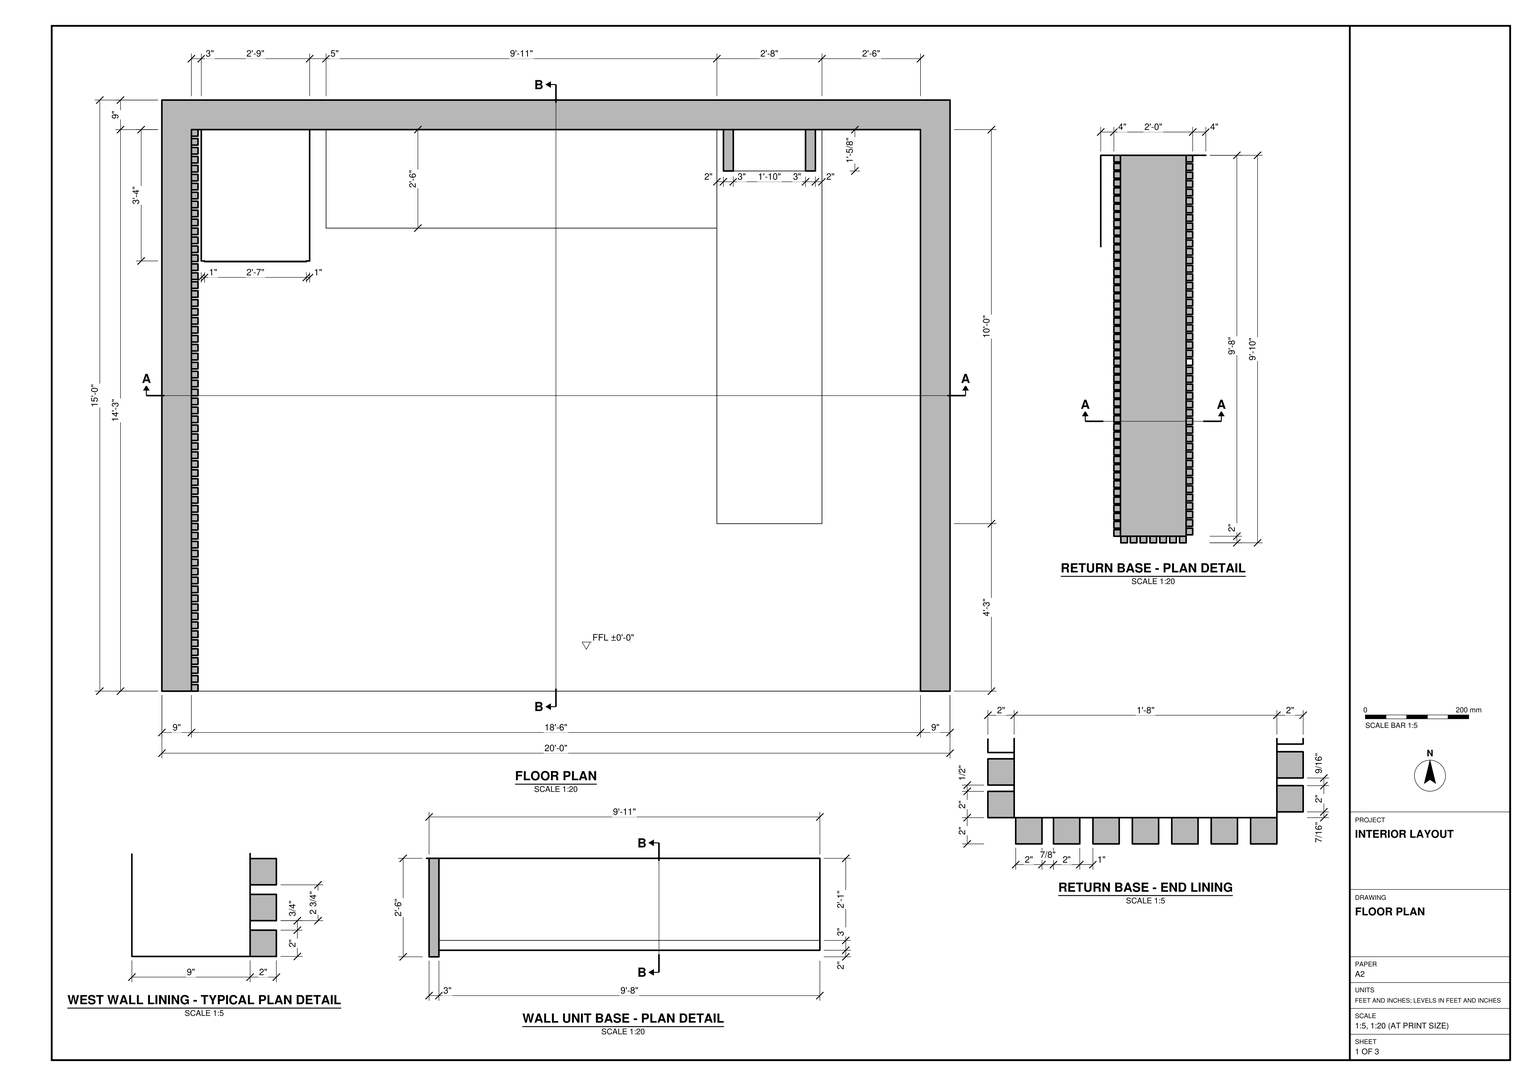
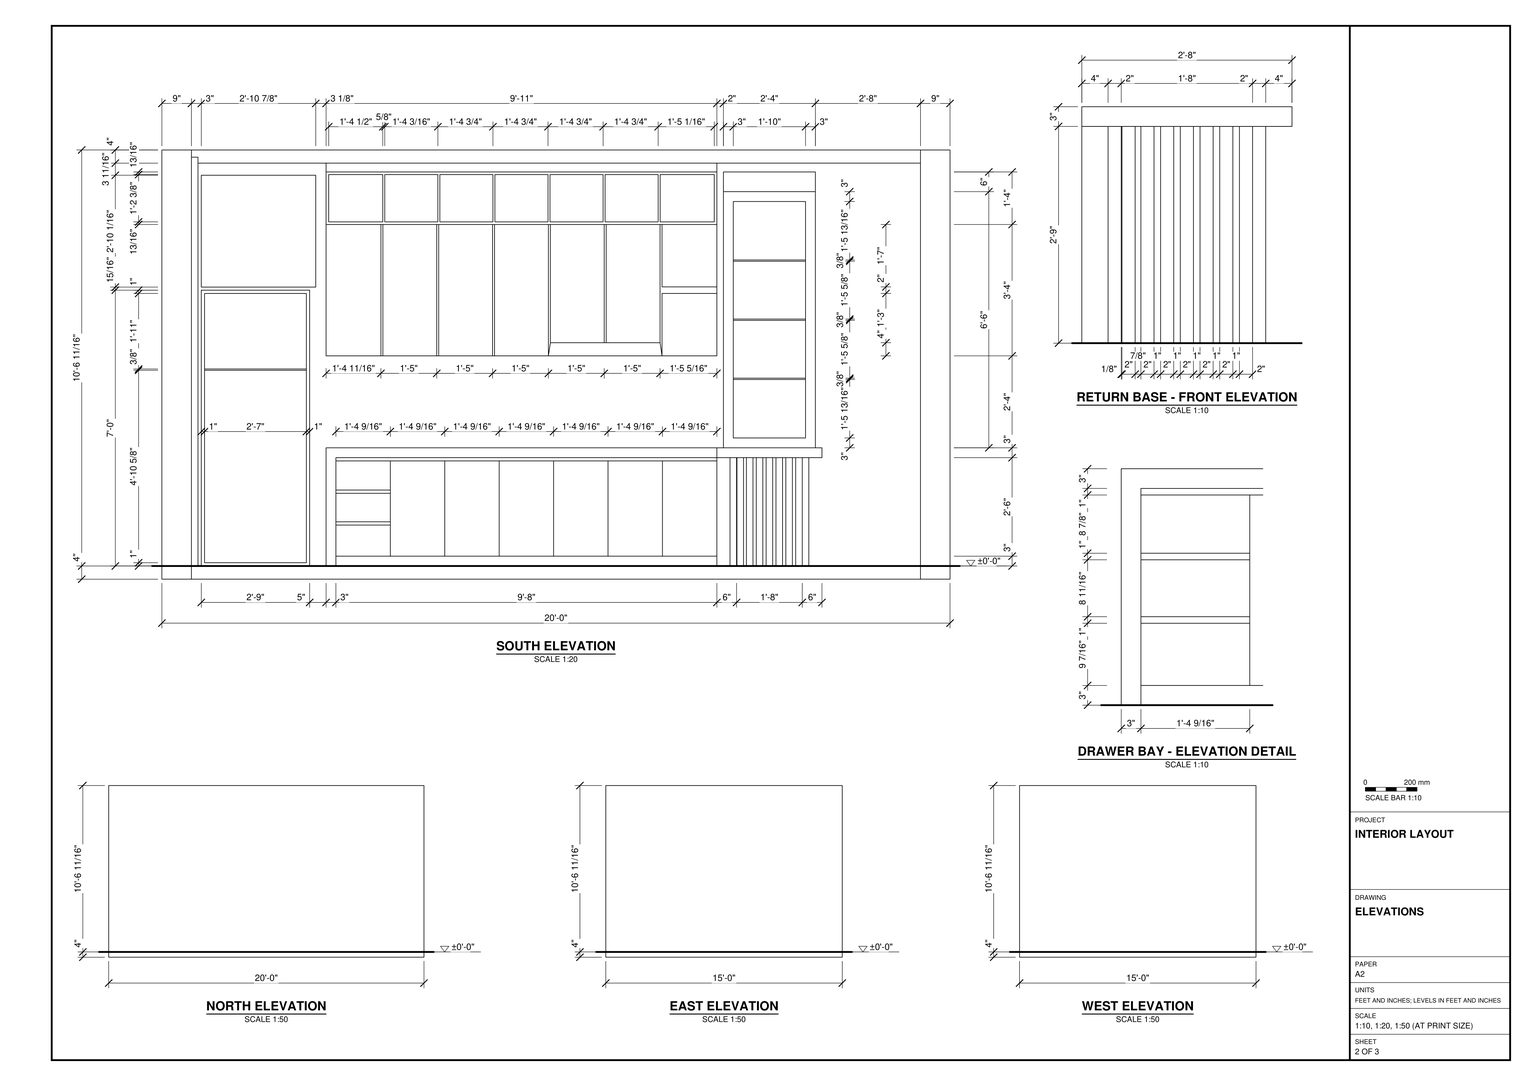
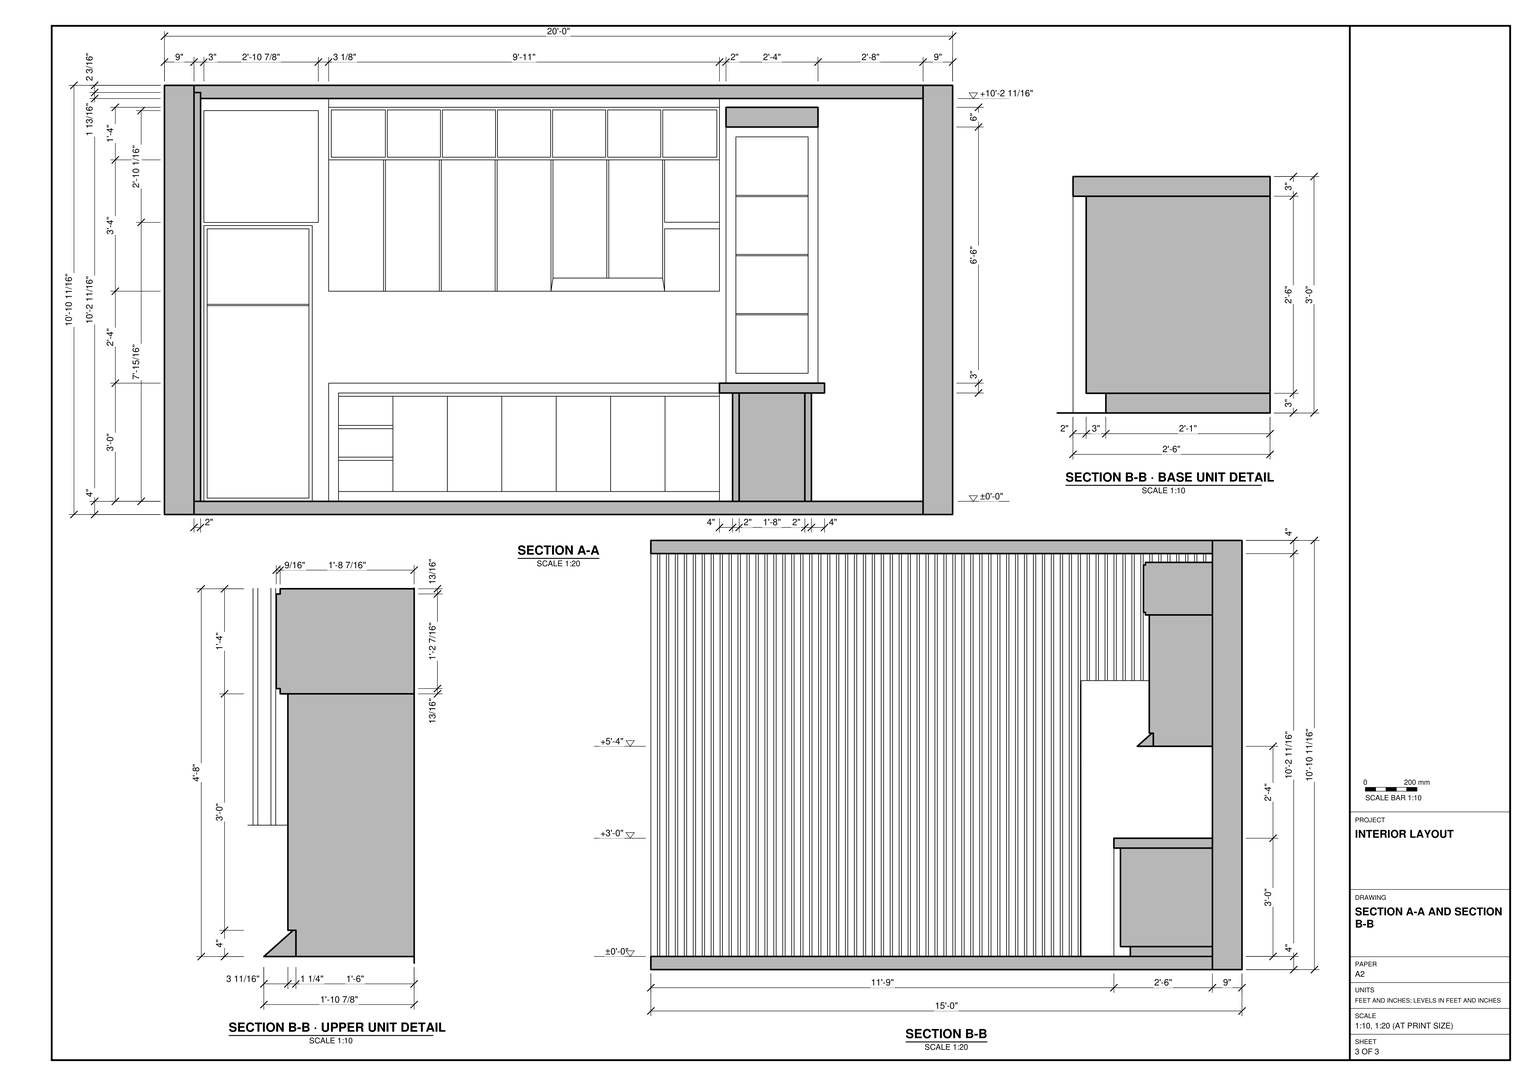
Build the single-level kitchen interior in SketchUp from task_files/diagram_01.pdf. Work in feet and inches. Set the finished floor at ±0'-0" and make the overall model 20'-0" wide, 15'-0" deep and 10'-10 11/16" high. Model the floor and overhead slabs, the 9" back and side walls, and the open front shown in plan. Line the inside of the west wall with the spaced vertical strips shown in the plan detail and section.

Use the south elevation to lay out the back wall. Place the tall unit and its overhead cupboard at the west end. Beside them, build the base cabinets with a drawer bay, divided fronts, a recessed plinth and a projecting countertop. Model the cupboards above the work surface in two tiers, following the changes in depth and lower-edge profile shown in section. At the right end, turn the counter into the room. Set its top over a narrower base with vertical strips along both sides and around the exposed end. Place the narrow shelving unit above the counter where the return meets the back wall.

Keep shell elements and each furniture or joinery piece in separate groups or components. Use components for repeated parts such as lining strips and cabinet fronts. Decor and loose items may be any suitable library components. Save one SketchUp model as output_files/kitchen_interior_with_a_slatted_counter_return.skp.

# SketchUp Ruby script. Lengths in inches.
U = 1.inch
M = Sketchup.active_model
def pt(a) = Geom::Point3d.new(a.map { |v| v * U })
def face(e, loops, mat)
  f = e.add_face(loops[0].map { |a| pt(a) })
  loops[1..].each { |l| e.add_face(l.map { |a| pt(a) }).erase! }
  f.material = f.back_material = mat if mat
  f
end
# faces: each face lists its corners as indices into pts; further lists are holes
def faces(e, pts, list, mat = nil) = list.each { |f| face(e, (f[0].is_a?(Array) ? f : [f]).map { |l| l.map { |i| pts[i] } }, mat) }
# xy, xz, yz: faces in a plane at the given z, y or x. An outline is a flat list of corners, or four numbers for a rectangle; further outlines are holes
def ring(l) = l.size == 4 ? [[l[0], l[1]], [l[2], l[1]], [l[2], l[3]], [l[0], l[3]]] : l.each_slice(2).to_a
def flat(e, list, mat, &to3) = list.each { |f| face(e, (f[0].is_a?(Array) ? f : [f]).map { |l| ring(l).map { |u, v| to3.(u, v) } }, mat) }
def xy(e, z, list, mat = nil) = flat(e, list, mat) { |x, y| [x, y, z] }
def xz(e, y, list, mat = nil) = flat(e, list, mat) { |x, z| [x, y, z] }
def yz(e, x, list, mat = nil) = flat(e, list, mat) { |y, z| [x, y, z] }
def lines(e, pts, list) = list.each { |a, b| e.add_line(pt(pts[a]), pt(pts[b])) }
# prism: a flat outline (further loops are holes) pulled along v
def prism(e, loops, v, mat = nil)
  f = face(e, loops, mat); d = Geom::Vector3d.new(v.map { |x| x * U })
  f.pushpull(f.normal.samedirection?(d) ? d.length : -d.length)
end
def box(e, o, s, mat = nil) = prism(e, [[o, [o[0] + s[0], o[1], o[2]], [o[0] + s[0], o[1] + s[1], o[2]], [o[0], o[1] + s[1], o[2]]]], [0, 0, s[2]], mat)
def at(x, y, z, deg = 0) = Geom::Transformation.translation(pt([x, y, z])) * Geom::Transformation.rotation(ORIGIN, Z_AXIS, deg.degrees)
def axes(o, x, y, z) = Geom::Transformation.new([*x, 0, *y, 0, *z, 0, *pt(o).to_a, 1])
def part(name) = M.definitions.add(name)
# library, detail: a bought-in or finely detailed component or shape, given as its bounding box
def library(name, o, s) = part(name).tap { |d| box(d.entities, o, s) }
def detail(e, o, s) = box(e.add_group.entities, o, s)
def put(e, d, t, mat = nil) = e.add_instance(d, t).tap { |i| i.material = mat if mat }
def group(e, t, mat = nil) = e.add_group.tap { |g| g.transformation = t; g.material = mat if mat }.entities
root = M.entities
M.materials.add("[0007_MistyRose]").color = [255, 228, 225]
M.materials.add("[0035_Tan]").color = [210, 180, 140]
M.materials.add("[0042_Sienna]").color = [160, 82, 45]
M.materials.add("[0043_SaddleBrown]").color = [139, 69, 19]
M.materials.add("[0131_Silver]").color = [192, 192, 192]
M.materials.add("[0134_DimGray]").color = [105, 105, 105]
M.materials.add("[0135_DarkGray]").color = [81, 81, 81]
M.materials.add("[0137_Black]").color = [0, 0, 0]
M.materials.add("[Carrera Marble]").color = [244, 244, 244]
M.materials.add("[Carrera Marble]1").color = [237, 237, 237]
M.materials.add("[Carrera Marble]2").color = [207, 207, 207]
M.materials.add("[Terrazzo Tile Accent]").color = [224, 221, 217]
M.materials.add("[Tile Various Tan]").color = [214, 196, 169]
M.materials.add("[Wood Bamboo]").color = [177, 105, 43]
c1 = part("Vertical timber slat")
box(c1.entities,[0,0,0],[2,2,124.5],"[Wood Bamboo]")
c2 = part("Horizontal counter slat")
box(c2.entities,[0,0,0],[2,33,2],"[Wood Bamboo]")
xy(root,-4,[[0,0,0,180,240,180,240,0,231,0,231,171,9,171,9,0]])
xy(root,0,[[12,131,45,171]])
xy(root,1,[[13,130.8,44,131]])
xy(root,59.6,[[13,130.8,44,131]])
xy(root,60,[[13,130.8,44,131]])
xy(root,64,[[117.7,148.11,152.3,153]],"[0135_DarkGray]")
xy(root,68,[[118.3,152.59,151.7,153]])
xy(root,83,[[13,130.8,44,131]])
xy(root,84,[[12,131,45,171]],"[0134_DimGray]")
xy(root,104,[[50,150.6,169,171]])
xy(root,104.8,[[50.8,150,67.27,150.6],[67.87,150,84.04,150.6],[84.64,150,100.8125,150.6],[101.41,150,117.59,150.6],[118.1875,150,134.36,150.6],
  [134.96,150,151.13,150.6],[151.73,150,168.2,150.6]])
xy(root,119.2,[[50.8,150,67.27,150.6],[67.87,150,84.04,150.6],[84.64,150,100.8125,150.6],[101.41,150,117.59,150.6],[118.1875,150,134.36,150.6],
  [134.96,150,151.13,150.6],[151.73,150,168.2,150.6]])
xy(root,120,[[50,150.6,169,171]])
xy(root,126.6875,[[0,0,9,0,9,171,231,171,231,0,240,0,240,180,0,180]])
xz(root,0,[[0,-4,9,126.6875],[231,-4,240,126.6875]])
xz(root,130.8,[[13,1,44,59.6],[13,60,44,83]],"[0131_Silver]")
xz(root,131,[[[12,0,45,84],[13,1,44,83]],[13,59.6,44,60]],"[0134_DimGray]")
xz(root,150,[[50.8,104.8,67.27,119.2],[67.87,104.8,84.04,119.2],[84.64,104.8,100.8125,119.2],[101.41,104.8,117.59,119.2],[118.1875,104.8,134.36,119.2],
  [134.96,104.8,151.13,119.2],[151.73,104.8,168.2,119.2]],"[0035_Tan]")
xz(root,150.6,[[[50,104,169,120],[151.73,104.8,168.2,119.2],[50.8,104.8,67.27,119.2],[118.1875,104.8,134.36,119.2],[84.64,104.8,100.8125,119.2],[101.41,104.8,117.59,119.2],[67.87,104.8,84.04,119.2],[134.96,104.8,151.13,119.2]]],"[0042_Sienna]")
xz(root,153,[[117.7,64,118.3,68,151.7,68,152.3,64]])
xz(root,171,[[[9,-4,12,-4,12,84,45,84,45,-4,231,-4,231,126.6875,169,126.6875,169,104,50,104,50,126.6875,9,126.6875],[174,93.2,196,111],[174,39,196,56.8],[174,75.2,196,92.8],[174,57.2,196,74.8]],[12,-4,45,84],[50,104,169,120],[50,120,169,126.6875]])
xz(root,171,[[174,39,196,56.8],[174,57.2,196,74.8],[174,75.2,196,92.8],[174,93.2,196,111]],"[Wood Bamboo]")
xz(root,180,[[0,-4,240,126.6875]])
yz(root,0,[[0,-4,180,126.6875]])
yz(root,9,[[0,-4,171,126.6875]])
yz(root,12,[[131,0,171,84]],"[0134_DimGray]")
yz(root,13,[[130.8,1,131,59.6],[130.8,60,131,83]])
yz(root,44,[[130.8,1,131,59.6],[130.8,60,131,83]])
yz(root,45,[[131,0,171,84]],"[0134_DimGray]")
yz(root,50,[[150.6,104,171,120]])
yz(root,50.8,[[150,104.8,150.6,119.2]])
yz(root,67.27,[[150,104.8,150.6,119.2]])
yz(root,67.87,[[150,104.8,150.6,119.2]])
yz(root,84.04,[[150,104.8,150.6,119.2]])
yz(root,84.64,[[150,104.8,150.6,119.2]])
yz(root,100.8125,[[150,104.8,150.6,119.2]])
yz(root,101.41,[[150,104.8,150.6,119.2]])
yz(root,117.59,[[150,104.8,150.6,119.2]])
yz(root,118.1875,[[150,104.8,150.6,119.2]])
yz(root,134.36,[[150,104.8,150.6,119.2]])
yz(root,134.96,[[150,104.8,150.6,119.2]])
yz(root,151.13,[[150,104.8,150.6,119.2]])
yz(root,151.73,[[150,104.8,150.6,119.2]])
yz(root,168.2,[[150,104.8,150.6,119.2]])
yz(root,169,[[150.6,104,171,120]])
yz(root,231,[[0,-4,171,126.6875]])
yz(root,240,[[0,-4,180,126.6875]])
p = [[151.7,152.59,68],[118.3,152.59,68],[117.7,148.11,64],[152.3,148.11,64],[118.3,153,68],[117.7,153,64],
  [152.3,153,64],[151.7,153,68]]
faces(root,p,[[0,1,2,3],[4,5,2,1],[6,7,0,3]],"[0135_DarkGray]")
put(root,c1,at(9,169,0))
put(root,c1,at(9,166.27,0))
put(root,c1,at(9,163.55,0))
put(root,c1,at(9,160.82,0))
put(root,c1,at(9,158.1,0))
put(root,c1,at(9,155.37,0))
put(root,c1,at(9,152.65,0))
put(root,c1,at(9,149.92,0))
put(root,c1,at(9,147.19,0))
put(root,c1,at(9,144.47,0))
put(root,c1,at(9,141.74,0))
put(root,c1,at(9,139.02,0))
put(root,c1,at(9,136.29,0))
put(root,c1,at(9,133.56,0))
put(root,c1,at(9,130.84,0))
put(root,c1,at(9,128.11,0))
put(root,c1,at(9,125.39,0))
put(root,c1,at(9,122.66,0))
put(root,c1,at(9,119.94,0))
put(root,c1,at(9,117.21,0))
put(root,c1,at(9,114.48,0))
put(root,c1,at(9,111.76,0))
put(root,c1,at(9,109.03,0))
put(root,c1,at(9,106.31,0))
put(root,c1,at(9,103.58,0))
put(root,c1,at(9,100.85,0))
put(root,c1,at(9,98.13,0))
put(root,c1,at(9,95.4,0))
put(root,c1,at(9,92.68,0))
put(root,c1,at(9,89.95,0))
put(root,c1,at(9,87.23,0))
put(root,c1,at(9,84.5,0))
put(root,c1,at(9,81.77,0))
put(root,c1,at(9,79.05,0))
put(root,c1,at(9,76.32,0))
put(root,c1,at(9,73.6,0))
put(root,c1,at(9,70.87,0))
put(root,c1,at(9,68.15,0))
put(root,c1,at(9,65.42,0))
put(root,c1,at(9,62.69,0))
put(root,c1,at(9,59.97,0))
put(root,c1,at(9,57.24,0))
put(root,c1,at(9,54.52,0))
put(root,c1,at(9,51.79,0))
put(root,c1,at(9,49.06,0))
put(root,c1,at(9,46.34,0))
put(root,c1,at(9,43.61,0))
put(root,c1,at(9,40.89,0))
put(root,c1,at(9,38.16,0))
put(root,c1,at(9,35.44,0))
put(root,c1,at(9,32.71,0))
put(root,c1,at(9,29.98,0))
put(root,c1,at(9,27.26,0))
put(root,c1,at(9,24.53,0))
put(root,c1,at(9,21.81,0))
put(root,c1,at(9,19.08,0))
put(root,c1,at(9,16.35,0))
put(root,c1,at(9,13.63,0))
put(root,c1,at(9,10.9,0))
put(root,c1,at(9,8.18,0))
put(root,c1,at(9,5.45,0))
put(root,c1,at(9,2.73,0))
put(root,c1,at(9,0,0))
put(root,c2,axes([173,171,0],[1,0,0],[0,0,1],[0,-1,0]))
put(root,c2,axes([173,168.52,0],[1,0,0],[0,0,1],[0,-1,0]))
put(root,c2,axes([173,166.04,0],[1,0,0],[0,0,1],[0,-1,0]))
put(root,c2,axes([173,163.57,0],[1,0,0],[0,0,1],[0,-1,0]))
put(root,c2,axes([173,161.09,0],[1,0,0],[0,0,1],[0,-1,0]))
put(root,c2,axes([173,158.61,0],[1,0,0],[0,0,1],[0,-1,0]))
put(root,c2,axes([173,156.13,0],[1,0,0],[0,0,1],[0,-1,0]))
put(root,c2,axes([173,153.65,0],[1,0,0],[0,0,1],[0,-1,0]))
put(root,c2,axes([173,151.17,0],[1,0,0],[0,0,1],[0,-1,0]))
put(root,c2,axes([173,148.7,0],[1,0,0],[0,0,1],[0,-1,0]))
put(root,c2,axes([173,146.22,0],[1,0,0],[0,0,1],[0,-1,0]))
put(root,c2,axes([173,143.74,0],[1,0,0],[0,0,1],[0,-1,0]))
put(root,c2,axes([173,141.26,0],[1,0,0],[0,0,1],[0,-1,0]))
put(root,c2,axes([173,138.78,0],[1,0,0],[0,0,1],[0,-1,0]))
put(root,c2,axes([173,136.3,0],[1,0,0],[0,0,1],[0,-1,0]))
put(root,c2,axes([173,133.83,0],[1,0,0],[0,0,1],[0,-1,0]))
put(root,c2,axes([173,131.35,0],[1,0,0],[0,0,1],[0,-1,0]))
put(root,c2,axes([173,128.87,0],[1,0,0],[0,0,1],[0,-1,0]))
put(root,c2,axes([173,126.39,0],[1,0,0],[0,0,1],[0,-1,0]))
put(root,c2,axes([173,123.91,0],[1,0,0],[0,0,1],[0,-1,0]))
put(root,c2,axes([173,121.43,0],[1,0,0],[0,0,1],[0,-1,0]))
put(root,c2,axes([173,118.96,0],[1,0,0],[0,0,1],[0,-1,0]))
put(root,c2,axes([173,116.48,0],[1,0,0],[0,0,1],[0,-1,0]))
put(root,c2,axes([173,114,0],[1,0,0],[0,0,1],[0,-1,0]))
put(root,c2,axes([173,111.52,0],[1,0,0],[0,0,1],[0,-1,0]))
put(root,c2,axes([173,109.04,0],[1,0,0],[0,0,1],[0,-1,0]))
put(root,c2,axes([173,106.57,0],[1,0,0],[0,0,1],[0,-1,0]))
put(root,c2,axes([173,104.09,0],[1,0,0],[0,0,1],[0,-1,0]))
put(root,c2,axes([173,101.61,0],[1,0,0],[0,0,1],[0,-1,0]))
put(root,c2,axes([173,99.13,0],[1,0,0],[0,0,1],[0,-1,0]))
put(root,c2,axes([173,96.65,0],[1,0,0],[0,0,1],[0,-1,0]))
put(root,c2,axes([173,94.17,0],[1,0,0],[0,0,1],[0,-1,0]))
put(root,c2,axes([173,91.7,0],[1,0,0],[0,0,1],[0,-1,0]))
put(root,c2,axes([173,89.22,0],[1,0,0],[0,0,1],[0,-1,0]))
put(root,c2,axes([173,86.74,0],[1,0,0],[0,0,1],[0,-1,0]))
put(root,c2,axes([173,84.26,0],[1,0,0],[0,0,1],[0,-1,0]))
put(root,c2,axes([173,81.78,0],[1,0,0],[0,0,1],[0,-1,0]))
put(root,c2,axes([173,79.3,0],[1,0,0],[0,0,1],[0,-1,0]))
put(root,c2,axes([173,76.83,0],[1,0,0],[0,0,1],[0,-1,0]))
put(root,c2,axes([173,74.35,0],[1,0,0],[0,0,1],[0,-1,0]))
put(root,c2,axes([173,71.87,0],[1,0,0],[0,0,1],[0,-1,0]))
put(root,c2,axes([173,69.39,0],[1,0,0],[0,0,1],[0,-1,0]))
put(root,c2,axes([173,66.91,0],[1,0,0],[0,0,1],[0,-1,0]))
put(root,c2,axes([173,64.43,0],[1,0,0],[0,0,1],[0,-1,0]))
put(root,c2,axes([173,61.96,0],[1,0,0],[0,0,1],[0,-1,0]))
put(root,c2,axes([173,59.48,0],[1,0,0],[0,0,1],[0,-1,0]))
put(root,c2,axes([173,57,0],[1,0,0],[0,0,1],[0,-1,0]))
put(root,c2,axes([175.12,55,0],[1,0,0],[0,0,1],[0,-1,0]))
put(root,c2,axes([177.99,55,0],[1,0,0],[0,0,1],[0,-1,0]))
put(root,c2,axes([181,55,0],[1,0,0],[0,0,1],[0,-1,0]))
put(root,c2,axes([184,55,0],[1,0,0],[0,0,1],[0,-1,0]))
put(root,c2,axes([187,55,0],[1,0,0],[0,0,1],[0,-1,0]))
put(root,c2,axes([190,55,0],[1,0,0],[0,0,1],[0,-1,0]))
put(root,c2,axes([193,55,0],[1,0,0],[0,0,1],[0,-1,0]))
put(root,c2,axes([195,171,0],[1,0,0],[0,0,1],[0,-1,0]))
put(root,c2,axes([195,168.42,0],[1,0,0],[0,0,1],[0,-1,0]))
put(root,c2,axes([195,165.84,0],[1,0,0],[0,0,1],[0,-1,0]))
put(root,c2,axes([195,163.26,0],[1,0,0],[0,0,1],[0,-1,0]))
put(root,c2,axes([195,160.68,0],[1,0,0],[0,0,1],[0,-1,0]))
put(root,c2,axes([195,158.1,0],[1,0,0],[0,0,1],[0,-1,0]))
put(root,c2,axes([195,155.51,0],[1,0,0],[0,0,1],[0,-1,0]))
put(root,c2,axes([195,152.93,0],[1,0,0],[0,0,1],[0,-1,0]))
put(root,c2,axes([195,150.35,0],[1,0,0],[0,0,1],[0,-1,0]))
put(root,c2,axes([195,147.77,0],[1,0,0],[0,0,1],[0,-1,0]))
put(root,c2,axes([195,145.19,0],[1,0,0],[0,0,1],[0,-1,0]))
put(root,c2,axes([195,142.61,0],[1,0,0],[0,0,1],[0,-1,0]))
put(root,c2,axes([195,140.03,0],[1,0,0],[0,0,1],[0,-1,0]))
put(root,c2,axes([195,137.45,0],[1,0,0],[0,0,1],[0,-1,0]))
put(root,c2,axes([195,134.87,0],[1,0,0],[0,0,1],[0,-1,0]))
put(root,c2,axes([195,132.29,0],[1,0,0],[0,0,1],[0,-1,0]))
put(root,c2,axes([195,129.7,0],[1,0,0],[0,0,1],[0,-1,0]))
put(root,c2,axes([195,127.125,0],[1,0,0],[0,0,1],[0,-1,0]))
put(root,c2,axes([195,124.54,0],[1,0,0],[0,0,1],[0,-1,0]))
put(root,c2,axes([195,121.96,0],[1,0,0],[0,0,1],[0,-1,0]))
put(root,c2,axes([195,119.38,0],[1,0,0],[0,0,1],[0,-1,0]))
put(root,c2,axes([195,116.8,0],[1,0,0],[0,0,1],[0,-1,0]))
put(root,c2,axes([195,114.22,0],[1,0,0],[0,0,1],[0,-1,0]))
put(root,c2,axes([195,111.64,0],[1,0,0],[0,0,1],[0,-1,0]))
put(root,c2,axes([195,109.06,0],[1,0,0],[0,0,1],[0,-1,0]))
put(root,c2,axes([195,106.48,0],[1,0,0],[0,0,1],[0,-1,0]))
put(root,c2,axes([195,103.89,0],[1,0,0],[0,0,1],[0,-1,0]))
put(root,c2,axes([195,101.3125,0],[1,0,0],[0,0,1],[0,-1,0]))
put(root,c2,axes([195,98.73,0],[1,0,0],[0,0,1],[0,-1,0]))
put(root,c2,axes([195,96.15,0],[1,0,0],[0,0,1],[0,-1,0]))
put(root,c2,axes([195,93.57,0],[1,0,0],[0,0,1],[0,-1,0]))
put(root,c2,axes([195,90.99,0],[1,0,0],[0,0,1],[0,-1,0]))
put(root,c2,axes([195,88.41,0],[1,0,0],[0,0,1],[0,-1,0]))
put(root,c2,axes([195,85.83,0],[1,0,0],[0,0,1],[0,-1,0]))
put(root,c2,axes([195,83.25,0],[1,0,0],[0,0,1],[0,-1,0]))
put(root,c2,axes([195,80.67,0],[1,0,0],[0,0,1],[0,-1,0]))
put(root,c2,axes([195,78.09,0],[1,0,0],[0,0,1],[0,-1,0]))
put(root,c2,axes([195,75.5,0],[1,0,0],[0,0,1],[0,-1,0]))
put(root,c2,axes([195,72.92,0],[1,0,0],[0,0,1],[0,-1,0]))
put(root,c2,axes([195,70.34,0],[1,0,0],[0,0,1],[0,-1,0]))
put(root,c2,axes([195,67.76,0],[1,0,0],[0,0,1],[0,-1,0]))
put(root,c2,axes([195,65.18,0],[1,0,0],[0,0,1],[0,-1,0]))
put(root,c2,axes([195,62.6,0],[1,0,0],[0,0,1],[0,-1,0]))
put(root,c2,axes([195,60.02,0],[1,0,0],[0,0,1],[0,-1,0]))
put(root,c2,axes([195,57.4375,0],[1,0,0],[0,0,1],[0,-1,0]))
g1 = group(root,at(50,143,0))
xy(g1,0,[[0,-2,3,28]],"[Carrera Marble]1")
xy(g1,33,[[3,-2,119,28]],"[Carrera Marble]1")
xy(g1,36,[[0,-2,119,28]],"[Carrera Marble]1")
xz(g1,-2,[[0,0,3,0,3,33,119,33,119,36,0,36]],"[Carrera Marble]1")
xz(g1,28,[[0,0,3,36],[3,33,117,36],[117,33,119,36]],"[Carrera Marble]1")
yz(g1,0,[[-2,0,28,36]],"[Carrera Marble]1")
yz(g1,3,[[-2,0,28,33]],"[Carrera Marble]1")
yz(g1,119,[[-2,33,28,36]],"[Carrera Marble]1")
g2 = group(root,at(169,51,0),"[Carrera Marble]")
box(g2,[0,0,33],[32,120,3])
g3 = group(root,at(50,143,-3))
xy(g3,6,[[3,0,119,28]])
xy(g3,36,[[3,0,119,28]])
xz(g3,0,[[3,6,19.57,15.47],[19.57,6,36.14,35],[36.14,6,52.71,35],[52.71,6,69.29,35],[69.29,6,85.86,35],
  [85.86,6,102.43,35],[102.43,6,119,35],[3,16.47,19.57,25.13],[3,26.13,19.57,35]],"[0035_Tan]")
xz(g3,0,[[3,15.47,19.57,16.47],[3,25.13,19.57,26.13],[3,35,119,36]],"[0043_SaddleBrown]")
xz(g3,28,[[3,6,119,36]])
yz(g3,3,[[0,6,28,36]])
yz(g3,119,[[0,6,28,36]])
g4 = group(root,at(169,51,-3))
box(g4,[6,4,3],[20,116,33],"[0007_MistyRose]")
g5 = group(root,at(50,143,-33))
box(g5,[3,3,33],[116,25,3],"[Carrera Marble]2")
g6 = group(root,at(171,159,36))
xy(g6,0,[[0,-0.6,28,12]],"[Wood Bamboo]")
xy(g6,3,[[3,-0.6,25,12]],"[Wood Bamboo]")
xy(g6,20.8,[[3,0,25,12]],"[Wood Bamboo]")
xy(g6,21.2,[[3,0,25,12]],"[Wood Bamboo]")
xy(g6,38.8,[[3,0,25,12]],"[Wood Bamboo]")
xy(g6,39.2,[[3,0,25,12]],"[Wood Bamboo]")
xy(g6,56.8,[[3,0,25,12]],"[Wood Bamboo]")
xy(g6,57.2,[[3,0,25,12]],"[Wood Bamboo]")
xy(g6,75,[[3,-0.6,25,12]],"[Wood Bamboo]")
xy(g6,78,[[0,-0.6,28,12]],"[Wood Bamboo]")
xz(g6,-0.6,[[[0,0,28,78],[3,3,25,75]]],"[0137_Black]")
xz(g6,0,[[3,20.8,25,21.2],[3,38.8,25,39.2],[3,56.8,25,57.2]],"[0137_Black]")
xz(g6,12,[[[0,0,28,78],[3,57.2,25,75],[3,3,25,20.8],[3,39.2,25,56.8],[3,21.2,25,38.8]]],"[Wood Bamboo]")
yz(g6,0,[[-0.6,0,12,78]],"[Wood Bamboo]")
yz(g6,3,[[-0.6,3,12,3,12,20.8,0,20.8,0,21.2,12,21.2,12,38.8,0,38.8,0,39.2,12,39.2,12,56.8,0,56.8,0,57.2,12,57.2,12,75,-0.6,75]],"[Wood Bamboo]")
yz(g6,25,[[-0.6,3,-0.6,75,12,75,12,57.2,0,57.2,0,56.8,12,56.8,12,39.2,0,39.2,0,38.8,12,38.8,12,21.2,0,21.2,0,20.8,12,20.8,12,3]],"[Wood Bamboo]")
yz(g6,28,[[-0.6,0,12,78]],"[Wood Bamboo]")
g7 = group(root,at(171,171,114))
box(g7,[0,-86.74,0],[28,86.74,6],"[Wood Bamboo]")
g8 = group(root,at(50,153,64))
xy(g8,0,[[102.3,-1.22,102.3,0,67.7,0,67.7,-0.6,51.3,-0.6,51.3,0,50.7,0,50.7,-0.6,34.3,-0.6,34.3,0,33.7,0,33.7,-0.6,17.3,-0.6,17.3,0,16.7,0,16.7,-0.6,0,-0.6,0,18,119,18,119,-1.22]])
xy(g8,4,[[68.3,-1.22,84.7,0],[85.3,-1.22,101.7,0]])
xy(g8,19,[[102.3,-1.22,119,0]])
xy(g8,21,[[102.3,-1.22,119,0]])
xy(g8,40,[[68.3,-1.22,84.7,-1.22,84.7,0,85.3,0,85.3,-1.22,101.7,-1.22,101.7,0,102.3,0,102.3,-1.22,119,-1.22,119,18,0,18,0,-0.6,16.7,-0.6,16.7,0,17.3,0,17.3,-0.6,33.7,-0.6,33.7,0,34.3,0,34.3,-0.6,50.7,-0.6,50.7,0,51.3,0,51.3,-0.6,67.7,-0.6,67.7,0,68.3,0]])
xz(g8,-1.22,[[102.3,0,119,19],[68.3,4,84.7,40],[85.3,4,101.7,40],[102.3,21,119,40]],"[0035_Tan]")
xz(g8,-0.6,[[0,0,16.7,40],[17.3,0,33.7,40],[34.3,0,50.7,40],[51.3,0,67.7,40]],"[0035_Tan]")
xz(g8,0,[[16.7,0,17.3,40],[33.7,0,34.3,40],[50.7,0,51.3,40]])
xz(g8,0,[[67.7,0,102.3,0,102.3,19,119,19,119,21,102.3,21,102.3,40,101.7,40,101.7,4,85.3,4,85.3,40,84.7,40,84.7,4,68.3,4,68.3,40,67.7,40]],"[0042_Sienna]")
xz(g8,18,[[0,0,119,40]])
yz(g8,0,[[-0.6,0,18,40]])
yz(g8,16.7,[[-0.6,0,0,40]])
yz(g8,17.3,[[-0.6,0,0,40]])
yz(g8,33.7,[[-0.6,0,0,40]])
yz(g8,34.3,[[-0.6,0,0,40]])
yz(g8,50.7,[[-0.6,0,0,40]])
yz(g8,51.3,[[-0.6,0,0,40]])
yz(g8,67.7,[[-0.6,0,0,40]])
yz(g8,68.3,[[-1.22,4,0,40]])
yz(g8,84.7,[[-1.22,4,0,40]])
yz(g8,85.3,[[-1.22,4,0,40]])
yz(g8,101.7,[[-1.22,4,0,40]])
yz(g8,102.3,[[-1.22,0,0,19],[-1.22,21,0,40]])
yz(g8,119,[[-1.22,0,18,0,18,40,-1.22,40,-1.22,21,0,21,0,19,-1.22,19]])
g9 = group(root,at(9,0,0),"[Terrazzo Tile Accent]")
xy(g9,-4,[[0,0,222,171]])
xy(g9,0,[[0,0,222,171]])
xz(g9,0,[[0,-4,222,0]],"[Tile Various Tan]")
xz(g9,171,[[0,-4,36,0],[36,-4,37,0],[37,-4,156,0],[156,-4,160,0],[160,-4,192,0],
  [192,-4,222,0]])
yz(g9,0,[[0,-4,171,0]])
yz(g9,222,[[0,-4,171,0]])
g10 = group(root,at(9,0,122.6875))
prism(g10,[[[2,0,0],[222,0,0],[222,0,4],[0,0,4],[0,0,1.8125],[2,0,1.8125]]],[0,171,0])
g11 = group(root,at(12,171,84.93))
xy(g11,0,[[0,-18.6,34.85,0]],"[Wood Bamboo]")
xy(g11,34.07,[[0,-18.6,34.85,0]],"[Wood Bamboo]")
xz(g11,-18.6,[[0,0,34.85,34.07]])
xz(g11,0,[[0,0,34.85,34.07]],"[Wood Bamboo]")
yz(g11,0,[[-18.6,0,0,34.07]],"[Wood Bamboo]")
yz(g11,34.85,[[-18.6,0,0,34.07]],"[Wood Bamboo]")
